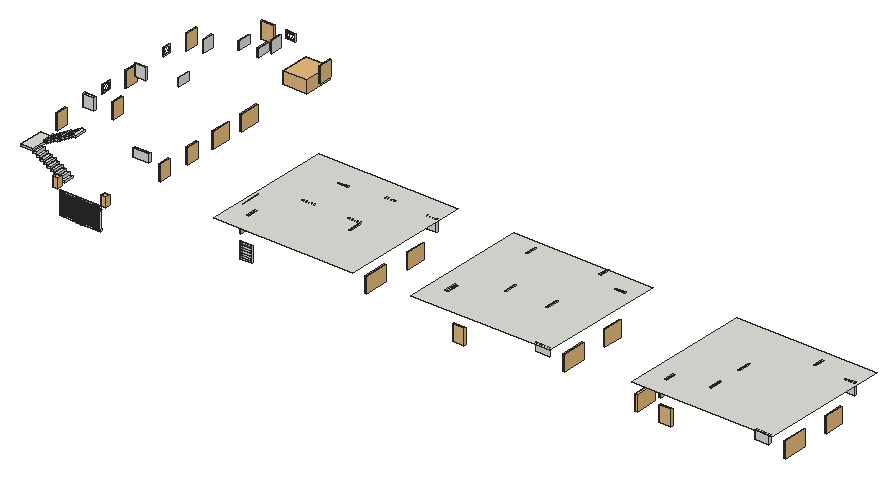
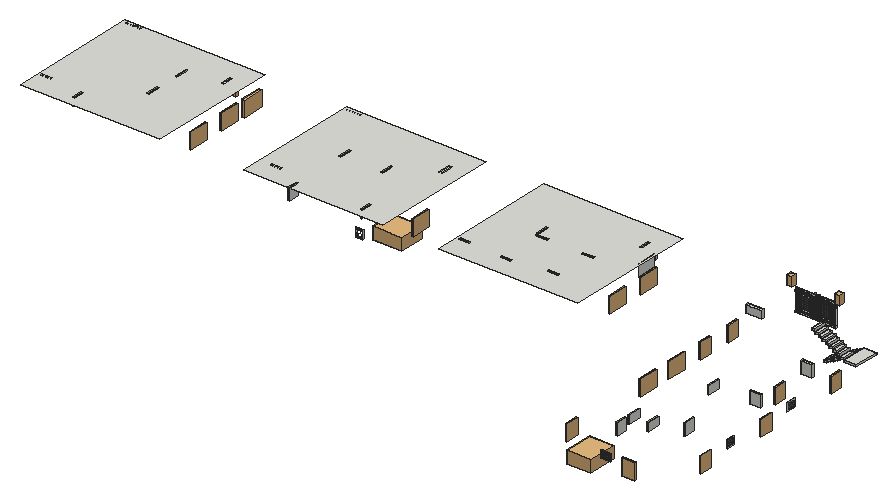
# SketchUp Ruby script. Lengths in inches.
U = 1.inch
M = Sketchup.active_model
def pt(a) = Geom::Point3d.new(a.map { |v| v * U })
def face(e, loops, mat)
  f = e.add_face(loops[0].map { |a| pt(a) })
  loops[1..].each { |l| e.add_face(l.map { |a| pt(a) }).erase! }
  f.material = f.back_material = mat if mat
  f
end
# faces: each face lists its corners as indices into pts; further lists are holes
def faces(e, pts, list, mat = nil) = list.each { |f| face(e, (f[0].is_a?(Array) ? f : [f]).map { |l| l.map { |i| pts[i] } }, mat) }
# xy, xz, yz: faces in a plane at the given z, y or x. An outline is a flat list of corners, or four numbers for a rectangle; further outlines are holes
def ring(l) = l.size == 4 ? [[l[0], l[1]], [l[2], l[1]], [l[2], l[3]], [l[0], l[3]]] : l.each_slice(2).to_a
def flat(e, list, mat, &to3) = list.each { |f| face(e, (f[0].is_a?(Array) ? f : [f]).map { |l| ring(l).map { |u, v| to3.(u, v) } }, mat) }
def xy(e, z, list, mat = nil) = flat(e, list, mat) { |x, y| [x, y, z] }
def xz(e, y, list, mat = nil) = flat(e, list, mat) { |x, z| [x, y, z] }
def yz(e, x, list, mat = nil) = flat(e, list, mat) { |y, z| [x, y, z] }
def lines(e, pts, list) = list.each { |a, b| e.add_line(pt(pts[a]), pt(pts[b])) }
# prism: a flat outline (further loops are holes) pulled along v
def prism(e, loops, v, mat = nil)
  f = face(e, loops, mat); d = Geom::Vector3d.new(v.map { |x| x * U })
  f.pushpull(f.normal.samedirection?(d) ? d.length : -d.length)
end
def box(e, o, s, mat = nil) = prism(e, [[o, [o[0] + s[0], o[1], o[2]], [o[0] + s[0], o[1] + s[1], o[2]], [o[0], o[1] + s[1], o[2]]]], [0, 0, s[2]], mat)
def at(x, y, z, deg = 0) = Geom::Transformation.translation(pt([x, y, z])) * Geom::Transformation.rotation(ORIGIN, Z_AXIS, deg.degrees)
def axes(o, x, y, z) = Geom::Transformation.new([*x, 0, *y, 0, *z, 0, *pt(o).to_a, 1])
def part(name) = M.definitions.add(name)
# library, detail: a bought-in or finely detailed component or shape, given as its bounding box
def library(name, o, s) = part(name).tap { |d| box(d.entities, o, s) }
def detail(e, o, s) = box(e.add_group.entities, o, s)
def put(e, d, t, mat = nil) = e.add_instance(d, t).tap { |i| i.material = mat if mat }
def group(e, t, mat = nil) = e.add_group.tap { |g| g.transformation = t; g.material = mat if mat }.entities
root = M.entities
M.materials.add("[Color_000]").color = [255, 255, 255]
M.materials.add("[Color_C20]").color = [102, 91, 81]
M.materials.add("[Translucent_Glass_Gray]").color = [128, 128, 128]
M.materials["[Translucent_Glass_Gray]"].alpha = 0.5
c1 = library("Untitled+(2)",[-25.65,-58.99,0],[75.48,89.46,37.24])
c2 = library("Gate pull handle",[-0.01,0,0],[1.26,2.875,48])
c3 = part("Gate slat")
xy(c3.entities,0,[[0.39,114.16,6.3,114.17]])
xy(c3.entities,0,[[0.39,0,6.3,114.16]],"[Color_C20]")
xy(c3.entities,0.39,[[0.39,0,0.79,114.17],[0.98,0,2.07,114.17],[2.36,0,3.2,114.17],[3.59,0,4.37,114.17],[4.56,0,5.71,114.17],
  [5.91,0,6.3,114.17]],"[Color_C20]")
xy(c3.entities,0.79,[[0.39,0,0.79,114.17],[0.98,0,2.07,114.17],[2.36,0,3.2,114.17],[3.59,0,4.37,114.17],[4.56,0,5.71,114.17],
  [5.91,0,6.3,114.17]],"[Color_C20]")
xy(c3.entities,0.99,[[1.13,0,1.21,114.16],[1.87,0,1.94,114.16],[2.61,0,2.68,114.16],[3.35,0,3.42,114.16],[4.08,0,4.16,114.16],
  [4.82,0,4.9,114.16],[5.5625,0,5.63,114.16],[6.3,0,6.37,114.16]],"[Color_C20]")
xy(c3.entities,1.18,[[0.39,114.16,3.35,114.17],[3.35,114.16,6.3,114.17]])
xy(c3.entities,1.18,[[0.39,0,1.13,114.16],[1.21,0,1.87,114.16],[1.94,0,2.61,114.16],[2.68,0,3.35,114.16],[3.42,0,4.08,114.16],
  [4.16,0,4.82,114.16],[4.9,0,5.5625,114.16],[5.63,0,6.3,114.16]],"[Color_C20]")
xz(c3.entities,0,[[[0.39,0,6.3,0,6.3,0.39,5.91,0.39,5.91,0.79,6.3,0.79,6.3,1.18,5.63,1.18,5.63,0.99,5.5625,0.99,5.5625,1.18,4.9,1.18,4.9,0.99,4.82,0.99,4.82,1.18,4.16,1.18,4.16,0.99,4.08,0.99,4.08,1.18,3.42,1.18,3.42,0.99,3.35,0.99,3.35,1.18,2.68,1.18,2.68,0.99,2.61,0.99,2.61,1.18,1.94,1.18,1.94,0.99,1.87,0.99,1.87,1.18,1.21,1.18,1.21,0.99,1.13,0.99,1.13,1.18,0.39,1.18,0.39,0.79,0.79,0.79,0.79,0.39,0.39,0.39],[4.56,0.39,5.71,0.79],[0.98,0.39,2.07,0.79],[2.36,0.39,3.2,0.79],[3.59,0.39,4.37,0.79]],[6.3,0.99,6.37,1.18]],"[Color_C20]")
xz(c3.entities,114.16,[[1.13,0.99,1.21,1.18],[1.87,0.99,1.94,1.18],[2.61,0.99,2.68,1.18],[3.35,0.99,3.42,1.18],[4.08,0.99,4.16,1.18],
  [4.82,0.99,4.9,1.18],[5.5625,0.99,5.63,1.18]],"[Color_C20]")
xz(c3.entities,114.17,[[[0.39,0,0.39,0.39,0.79,0.39,0.79,0.79,0.39,0.79,0.39,1.18,6.3,1.18,6.3,0.79,5.91,0.79,5.91,0.39,6.3,0.39,6.3,0],[4.56,0.39,5.71,0.79],[0.98,0.39,2.07,0.79],[2.36,0.39,3.2,0.79],[3.59,0.39,4.37,0.79]]],"[Color_C20]")
yz(c3.entities,0.39,[[114.16,0,114.17,0.39],[114.16,0.79,114.17,1.18]])
yz(c3.entities,0.39,[[0,0,114.16,0.39],[0,0.79,114.16,1.18]],"[Color_C20]")
yz(c3.entities,0.79,[[0,0.39,114.17,0.79]],"[Color_C20]")
yz(c3.entities,0.98,[[0,0.39,114.17,0.79]],"[Color_C20]")
yz(c3.entities,1.13,[[0,0.99,114.16,1.18]],"[Color_C20]")
yz(c3.entities,1.21,[[0,0.99,114.16,1.18]],"[Color_C20]")
yz(c3.entities,1.87,[[0,0.99,114.16,1.18]],"[Color_C20]")
yz(c3.entities,1.94,[[0,0.99,114.16,1.18]],"[Color_C20]")
yz(c3.entities,2.07,[[0,0.39,114.17,0.79]],"[Color_C20]")
yz(c3.entities,2.36,[[0,0.39,114.17,0.79]],"[Color_C20]")
yz(c3.entities,2.61,[[0,0.99,114.16,1.18]],"[Color_C20]")
yz(c3.entities,2.68,[[0,0.99,114.16,1.18]],"[Color_C20]")
yz(c3.entities,3.2,[[0,0.39,114.17,0.79]],"[Color_C20]")
yz(c3.entities,3.35,[[0,0.99,114.16,1.18]],"[Color_C20]")
yz(c3.entities,3.42,[[0,0.99,114.16,1.18]],"[Color_C20]")
yz(c3.entities,3.59,[[0,0.39,114.17,0.79]],"[Color_C20]")
yz(c3.entities,4.08,[[0,0.99,114.16,1.18]],"[Color_C20]")
yz(c3.entities,4.16,[[0,0.99,114.16,1.18]],"[Color_C20]")
yz(c3.entities,4.37,[[0,0.39,114.17,0.79]],"[Color_C20]")
yz(c3.entities,4.56,[[0,0.39,114.17,0.79]],"[Color_C20]")
yz(c3.entities,4.82,[[0,0.99,114.16,1.18]],"[Color_C20]")
yz(c3.entities,4.9,[[0,0.99,114.16,1.18]],"[Color_C20]")
yz(c3.entities,5.5625,[[0,0.99,114.16,1.18]],"[Color_C20]")
yz(c3.entities,5.63,[[0,0.99,114.16,1.18]],"[Color_C20]")
yz(c3.entities,5.71,[[0,0.39,114.17,0.79]],"[Color_C20]")
yz(c3.entities,5.91,[[0,0.39,114.17,0.79]],"[Color_C20]")
yz(c3.entities,6.3,[[114.16,0,114.17,0.39],[114.16,0.79,114.17,1.18]])
yz(c3.entities,6.3,[[0,0,114.16,0.39],[0,0.79,114.16,0.99],[0,0.99,114.16,1.18]],"[Color_C20]")
yz(c3.entities,6.37,[[0,0.99,114.16,1.18]],"[Color_C20]")
p = [[0,0,0],[0.39,0,0]]
lines(c3.entities,p,[[0,1]])
c4 = part("Vertical gate panel")
put(c4.entities,c3,axes([0,1.18,0],[3.67755,0,0],[0,0,2.40086],[0,-1,0]))
put(c4.entities,c3,axes([21.72,1.18,0],[3.67755,0,0],[0,0,2.40086],[0,-1,0]))
c5 = part("Group\#1")
prism(c5.entities,[[[0,0,0],[0,31.5,0],[11,31.5,0],[11,0,0],[2,0,0]]],[0,0,6])
c6 = library("Window with transom",[0,0,0],[5.2,55.12,70.87])
c7 = part("Group\#259")
p = [[0,43.31,5.11],[2.95,43.31,0],[2.95,0,0],[0,0,5.11]]
faces(c7.entities,p,[[0,1,2,3]],"[Translucent_Glass_Gray]")
c8 = part("Vwntilation+window (1)")
put(c8.entities,c7,at(43.48,1.97,32.29))
put(c8.entities,c7,at(43.48,1.97,26.38))
put(c8.entities,c7,at(43.48,1.97,20.48))
put(c8.entities,c7,at(43.48,1.97,14.57))
put(c8.entities,c7,at(43.48,1.97,8.67))
put(c8.entities,c7,at(43.48,1.97,2.76))
g1 = group(c8.entities,at(43.48,0,0))
prism(g1,[[[1.97,47.24,39.37],[1.97,0,39.37],[1.97,0,0],[1.97,47.24,0]],[[1.97,45.28,1.97],[1.97,1.97,1.97],[1.97,1.97,37.4],[1.97,45.28,37.4]]],[-1.97,0,0])
c9 = part("Group\#3")
box(c9.entities,[0,0,0],[11,37.5,6])
c10 = library("Group\#257",[0,0,0],[26.45,25.63,49.07])
xy(root,1.13,[[[260.49,22.66,324.4,26.05],[262.38,24.13,262.49,24.15,262.6,24.19,262.69,24.26,262.76,24.36,262.81,24.46,262.82,24.58,262.81,24.69,262.76,24.8,262.69,24.89,262.6,24.97,262.49,25.01,262.38,25.02,262.26,25.01,262.15,24.97,262.0625,24.89,261.99,24.8,261.95,24.69,261.93,24.58,261.95,24.46,261.99,24.36,262.0625,24.26,262.15,24.19,262.26,24.15]],[[324.65,22.66,387.35,25.83],[386.67,24.04,386.79,24.05,386.9,24.09,386.99,24.16,387.06,24.24,387.1,24.34,387.12,24.45,387.1,24.56,387.06,24.66,386.99,24.75,386.9,24.8125,386.79,24.85,386.67,24.87,386.56,24.85,386.45,24.8125,386.36,24.75,386.29,24.66,386.24,24.56,386.23,24.45,386.24,24.34,386.29,24.24,386.36,24.16,386.45,24.09,386.56,24.05]]],"[Color_000]")
xy(root,4.67,[[276.34,22.66,277.85,23.22],[277.85,22.66,309.42,23.22],[309.42,22.66,310.93,23.22],[338.12,22.66,339.63,23.18],[339.63,22.66,371.2,23.18],
  [371.2,22.66,372.71,23.18]])
xy(root,4.67,[[266.41,22.66,271.38,26.05],[271.38,22.66,276.34,26.05],[310.93,22.66,320.86,23.22],[328.1875,22.66,338.12,23.18],[372.71,22.66,377.67,25.83],
  [377.67,22.66,382.64,25.83],[328.1875,23.18,338.12,25.83],[339.63,23.18,371.2,25.83],[277.85,23.22,309.42,26.05],[310.93,23.22,320.86,26.05]],"[Color_000]")
xy(root,6,[[260.49,22.66,262.88,26.05],[386.17,22.66,387.35,25.83]],"[Color_000]")
xy(root,14.6,[[277.85,22.66,309.42,26.05],[339.63,22.66,371.2,25.83]],"[Color_000]")
xy(root,16.11,[[277.85,22.66,309.42,26.05],[339.63,22.66,371.2,25.83]],"[Color_000]")
xy(root,56.27,[[277.85,22.66,309.42,26.05],[339.63,22.66,371.2,25.83]],"[Color_000]")
xy(root,57.78,[[277.85,22.66,309.42,26.05],[339.63,22.66,371.2,25.83]],"[Color_000]")
xy(root,58.06,[[386.17,23.78,387.29,24.97],[261.76,23.86,262.88,25.14]],"[Color_000]")
xy(root,60.46,[[386.17,23.78,387.29,24.97],[261.76,23.86,262.88,25.14]],"[Color_000]")
xy(root,60.57,[[386.17,23.78,387.29,24.97],[387.29,23.78,389.6,24.97],[259.45,23.86,261.76,25.14],[261.76,23.86,262.88,25.14]],"[Color_000]")
xy(root,61.29,[[386.17,23.78,387.29,24.97],[387.29,23.78,389.6,24.97],[259.45,23.86,261.76,25.14],[261.76,23.86,262.88,25.14]],"[Color_000]")
xy(root,61.41,[[386.17,23.78,387.29,24.97],[261.76,23.86,262.88,25.14]],"[Color_000]")
xy(root,63.71,[[386.17,23.78,387.29,24.97],[261.76,23.86,262.88,25.14]],"[Color_000]")
xy(root,67.71,[[266.41,22.66,271.38,26.05],[271.38,22.66,276.34,26.05],[277.85,22.66,309.42,26.05],[310.93,22.66,320.86,26.05],[328.1875,22.66,338.12,25.83],
  [339.63,22.66,371.2,25.83],[372.71,22.66,377.67,25.83],[377.67,22.66,382.64,25.83]],"[Color_000]")
xy(root,71.24,[[262.88,22.66,324.4,26.05],[324.65,22.66,386.17,25.83]],"[Color_000]")
xy(root,120,[[692.13,78.48,1123.13,483.48],[1300.75,78.48,1731.75,474.48],[1983.63,78.48,2414.63,483.48]])
xz(root,22.66,[[[260.49,1.13,324.4,1.13,324.4,71.24,262.88,71.24,262.88,6,260.49,6],[266.41,4.67,320.86,67.71]],[[324.65,1.13,387.35,1.13,387.35,6,386.17,6,386.17,71.24,324.65,71.24],[328.1875,4.67,382.64,67.71]],[276.34,4.67,277.85,14.6],[309.42,4.67,310.93,14.6],[338.12,4.67,339.63,14.6],
  [371.2,4.67,372.71,14.6],[276.34,14.6,310.93,14.6,310.93,57.78,276.34,57.78,276.34,56.27,309.42,56.27,309.42,16.11,277.85,16.11,277.85,56.27,276.34,56.27],[338.12,14.6,372.71,14.6,372.71,56.27,371.2,56.27,371.2,16.11,339.63,16.11,339.63,56.27,372.71,56.27,372.71,57.78,338.12,57.78],[276.34,57.78,277.85,67.71],[309.42,57.78,310.93,67.71],
  [338.12,57.78,339.63,67.71],[371.2,57.78,372.71,67.71]],"[Color_000]")
xz(root,23.78,[[386.17,58.06,387.29,60.46],[386.17,60.57,389.6,61.29],[386.17,61.41,387.29,63.71]],"[Color_000]")
xz(root,23.86,[[261.76,58.06,262.88,60.46],[259.45,60.57,262.88,61.29],[261.76,61.41,262.88,63.71]],"[Color_000]")
xz(root,24.97,[[386.17,58.06,387.29,60.46],[386.17,60.57,387.29,60.85],[387.29,60.57,387.29,60.85,386.17,60.85,386.17,61.29,389.6,61.29,389.6,60.57],[386.17,61.41,387.29,63.71]],"[Color_000]")
xz(root,25.14,[[261.76,58.06,262.88,60.46],[259.45,60.57,259.45,61.29,262.88,61.29,262.88,60.85,261.76,60.85,261.76,60.57],[261.76,60.57,262.88,60.85],[261.76,61.41,262.88,63.71]],"[Color_000]")
xz(root,25.83,[[[324.65,1.13,324.65,71.24,386.17,71.24,386.17,6,387.35,6,387.35,1.13],[339.63,16.11,371.2,56.27],[372.71,4.67,382.64,67.71],[328.1875,4.67,338.12,67.71],[339.63,57.78,371.2,67.71],[339.63,4.67,371.2,14.6]]],"[Color_000]")
xz(root,26.05,[[[260.49,1.13,260.49,6,262.88,6,262.88,71.24,324.4,71.24,324.4,1.13],[277.85,16.11,309.42,56.27],[266.41,4.67,276.34,67.71],[310.93,4.67,320.86,67.71],[277.85,57.78,309.42,67.71],[277.85,4.67,309.42,14.6]]],"[Color_000]")
xz(root,87.48,[[1679.75,96,1722.75,120]])
yz(root,259.45,[[23.86,60.57,25.14,61.29]],"[Color_000]")
yz(root,260.49,[[22.66,1.13,26.05,6]],"[Color_000]")
yz(root,261.76,[[23.86,58.06,25.14,60.46],[23.86,61.41,25.14,63.71]],"[Color_000]")
yz(root,262.88,[[[22.66,6,26.05,71.24],[23.86,58.06,25.14,60.46],[23.86,61.41,25.14,63.71],[23.86,60.57,25.14,61.29]]],"[Color_000]")
yz(root,266.41,[[22.66,4.67,26.05,67.71]],"[Color_000]")
yz(root,276.34,[[22.66,4.67,26.05,14.6],[22.66,14.6,26.05,56.27],[22.66,56.27,26.05,57.78],[22.66,57.78,26.05,67.71]],"[Color_000]")
yz(root,277.85,[[22.66,4.67,26.05,14.6],[22.66,16.11,26.05,56.27],[22.66,57.78,26.05,67.71]],"[Color_000]")
yz(root,309.42,[[22.66,4.67,26.05,14.6],[22.66,16.11,26.05,56.27],[22.66,57.78,26.05,67.71]],"[Color_000]")
yz(root,310.93,[[22.66,4.67,26.05,14.6],[22.66,14.6,26.05,57.78],[22.66,57.78,26.05,67.71]],"[Color_000]")
yz(root,320.86,[[22.66,4.67,26.05,67.71]],"[Color_000]")
yz(root,324.4,[[22.66,1.13,26.05,71.24]],"[Color_000]")
yz(root,324.65,[[22.66,1.13,25.83,71.24]],"[Color_000]")
yz(root,328.1875,[[22.66,4.67,25.83,67.71]],"[Color_000]")
yz(root,338.12,[[22.66,4.67,25.83,14.6],[22.66,14.6,25.83,57.78],[22.66,57.78,25.83,67.71]],"[Color_000]")
yz(root,339.63,[[22.66,4.67,25.83,14.6],[22.66,16.11,25.83,56.27],[22.66,57.78,25.83,67.71]],"[Color_000]")
yz(root,371.2,[[22.66,4.67,25.83,14.6],[22.66,16.11,25.83,56.27],[22.66,57.78,25.83,67.71]],"[Color_000]")
yz(root,372.71,[[22.66,4.67,25.83,14.6],[22.66,14.6,25.83,56.27],[22.66,56.27,25.83,57.78],[22.66,57.78,25.83,67.71]],"[Color_000]")
yz(root,382.64,[[22.66,4.67,25.83,67.71]],"[Color_000]")
yz(root,386.17,[[[22.66,6,25.83,71.24],[23.78,58.06,23.78,60.46,24.97,60.46,24.97,60.57,23.78,60.57,23.78,61.29,24.97,61.29,24.97,58.06],[23.78,61.41,24.97,63.71]]],"[Color_000]")
yz(root,387.29,[[23.78,58.06,24.97,60.46],[23.78,61.41,24.97,63.71]],"[Color_000]")
yz(root,387.35,[[22.66,1.13,25.83,6]],"[Color_000]")
yz(root,701.13,[[178.48,84,239.48,120]])
p = [[373.33,23.18,4.67],[372.71,23.18,4.67],[375.83,23.18,67.7],[339.63,23.18,67.7],[371.19,23.18,58.15],[371.19,23.18,16.11],
  [273.22,23.22,67.7],[309.42,23.22,67.7],[275.72,23.22,4.67],[276.34,23.22,4.67],[277.86,23.22,58.15],[277.86,23.22,16.11],
  [324.4,22.66,1.13],[324.65,22.66,1.13],[262.88,25.14,60.57],[262.88,25.14,60.46]]
lines(root,p,[[0,1],[2,3],[4,5],[6,7],[8,9],[10,11],[12,13],[14,15]])
put(root,c1,at(303.23,921.85,0.9))
put(root,c2,axes([331.23,19.9,1.41],[-0.989,0,0],[0,0.96118,0],[0,0,1.45482]))
put(root,c2,axes([317.82,19.7,1.41],[0.989,0,0],[0,1.03,0],[0,0,1.45482]))
put(root,c4,axes([339.63,23.18,4.33],[0,0,0.23456],[0,0.21463,0],[0.11517,0,0]))
put(root,c4,axes([309.42,23.22,4.33],[0,0,0.23456],[0,0.23,0],[-0.11517,0,0]))
put(root,c3,axes([333.52,23.4375,4.67],[-0.84584,0,0],[0,0,0.5522],[0,-0.21463,0]))
put(root,c3,axes([383.03,23.4375,4.67],[-0.84584,0,0],[0,0,0.5522],[0,-0.21463,0]))
put(root,c3,axes([378.03,23.4375,4.67],[-0.84584,0,0],[0,0,0.5522],[0,-0.21463,0]))
put(root,c3,axes([338.51,23.4375,4.67],[-0.84584,0,0],[0,0,0.5522],[0,-0.21463,0]))
put(root,c3,axes([266.02,23.49,4.67],[0.84584,0,0],[0,0,0.5522],[0,-0.23,0]))
put(root,c3,axes([271.02,23.49,4.67],[0.84584,0,0],[0,0,0.5522],[0,-0.23,0]))
put(root,c3,axes([310.54,23.49,4.67],[0.84584,0,0],[0,0,0.5522],[0,-0.23,0]))
put(root,c3,axes([315.53,23.49,4.67],[0.84584,0,0],[0,0,0.5522],[0,-0.23,0]))
put(root,c1,at(1342.19,338.62,5.79,90))
put(root,c5,at(166,148.42,6))
put(root,c5,at(155,148.42,12))
put(root,c4,axes([339.625,23.18,15.98],[0,0,0.22998],[0,0.21463,0],[0.11517,0,0]))
put(root,c4,axes([309.43,23.22,15.98],[0,0,0.22998],[0,0.23,0],[-0.11517,0,0]))
put(root,c5,at(144,148.42,18))
put(root,c5,at(133,148.42,24))
put(root,c4,axes([339.625,23.18,25.97],[0,0,0.22998],[0,0.21463,0],[0.11517,0,0]))
put(root,c4,axes([309.43,23.22,25.97],[0,0,0.22998],[0,0.23,0],[-0.11517,0,0]))
put(root,c5,at(122,148.42,30))
put(root,c4,axes([339.63,23.18,35.96],[0,0,0.22998],[0,0.21463,0],[0.11517,0,0]))
put(root,c4,axes([309.42,23.22,35.96],[0,0,0.22998],[0,0.23,0],[-0.11517,0,0]))
put(root,c6,axes([1300.71,298.48,35.96],[1,0,0],[0,1.08857,0],[0,0,0.67733]))
put(root,c6,axes([1114.09,134.48,35.96],[1,0,0],[0,1.33894,0],[0,0,0.67733]))
put(root,c6,axes([1123.13,290.48,35.96],[-0.73939,0,0],[0,1.08857,0],[0,0,0.67733]))
put(root,c6,axes([29.96,564.92,35.96],[1,0,0],[0,0.70757,0],[0,0,0.67733]))
put(root,c6,axes([29.96,797.29,35.96],[1,0,0],[0,0.70757,0],[0,0,0.67733]))
put(root,c6,axes([380.96,874.91,35.96],[1,0,0],[0,0.70757,0],[0,0,0.67733]))
put(root,c6,axes([380.96,569.64,35.96],[1,0,0],[0,1.10381,0],[0,0,0.67733]))
put(root,c6,axes([380.96,459.92,35.96],[1,0,0],[0,1.10381,0],[0,0,0.67733]))
put(root,c6,axes([380.96,361.31,35.96],[1,0,0],[0,0.66512,0],[0,0,0.67733]))
put(root,c6,axes([380.96,255.61,35.96],[1,0,0],[0,0.66512,0],[0,0,0.67733]))
put(root,c6,axes([692.15,178.46,35.96],[1,0,0],[0,1.10671,0],[0,0,0.67733]))
put(root,c6,axes([692.15,298.48,35.96],[1,0,0],[0,1.10671,0],[0,0,0.67733]))
put(root,c6,axes([1987.4375,178.48,36],[1,0,0],[0,1.10671,0],[0,0,0.67733]))
put(root,c6,axes([1987.4375,298.48,36],[1,0,0],[0,1.08857,0],[0,0,0.67733]))
put(root,c6,axes([1983.63,88.48,36],[1.73182,0,0],[0,1.23371,0],[0,0,0.67733]))
put(root,c8,axes([773.13,142.97,36],[0,-1.3889,0],[0.762,0,0],[0,0,1.2192]))
put(root,c6,axes([30,296.72,36],[1,0,0],[0,0.65314,0],[0,0,0.67733]))
put(root,c6,axes([174,957.23,36],[0,1,0],[-0.70757,0,0],[0,0,0.67733]))
put(root,c6,axes([100.5,423.92,36],[1.23,0,0],[0,0.64389,0],[0,0,0.67733]))
put(root,c6,axes([1726.56,134.48,36],[1,0,0],[0,1.34257,0],[0,0,0.67733]))
put(root,c6,axes([1726.56,290.48,36],[1,0,0],[0,1.08857,0],[0,0,0.67733]))
put(root,c6,axes([2409.18,290.7,36],[1.05,0,0],[0,1.08458,0],[0,0,0.67733]))
put(root,c6,axes([2409.18,134.48,36],[1.05,0,0],[0,1.34257,0],[0,0,0.67733]))
put(root,c6,axes([1461.75,83.28,36],[0,1,0],[-0.65552,0,0],[0,0,0.67733]))
put(root,c6,axes([2100.63,83.28,36],[0,1,0],[-0.65552,0,0],[0,0,0.67733]))
put(root,c5,at(111,148.42,36))
put(root,c5,at(100,148.42,42))
put(root,c4,axes([339.63,23.18,45.95],[0,0,0.22998],[0,0.21463,0],[0.11517,0,0]))
put(root,c4,axes([309.42,23.22,45.95],[0,0,0.22998],[0,0.23,0],[-0.11517,0,0]))
put(root,c5,at(89,148.42,48))
put(root,c5,at(78,148.42,54))
put(root,c4,axes([339.63,23.18,57.18],[0,0,0.23456],[0,0.21463,0],[0.11517,0,0]))
put(root,c4,axes([309.42,23.22,57.18],[0,0,0.23456],[0,0.23,0],[-0.11517,0,0]))
put(root,c8,axes([94.49,732.63,60],[-1.3889,0,0],[0,-0.508,0],[0,0,0.6096]))
put(root,c8,axes([94.49,501.82,60],[-1.3889,0,0],[0,-0.635,0],[0,0,0.6096]))
g2 = group(root,at(39,148.42,60))
box(g2,[0,0,0],[39,78,6])
put(root,c8,axes([1359.6,538.97,60],[0,-1.3889,0],[0.51054,0,0],[0,0,0.6096]))
put(root,c8,axes([238.5,934.1,62.25],[0,0.61,0],[-0.635,0,0],[0,0,0.55235]))
put(root,c9,at(78,188.92,66))
put(root,c9,at(89,188.92,72))
put(root,c10,axes([241.95,20.69,74.85],[0.58,0,0],[0,0.58,0],[0,0,0.58]))
put(root,c10,axes([390.15,20.69,74.85],[0.58,0,0],[0,0.58,0],[0,0,0.58]))
put(root,c9,at(100,188.92,78))
g3 = group(root,at(121.5,749.42,0))
box(g3,[0,0,84],[4.5,33,36])
put(root,c9,at(111,188.92,84))
g4 = group(root,at(63,359.92,0))
box(g4,[0,0,84],[33,9,36])
g5 = group(root,at(67.5,555.92,0))
box(g5,[0,0,84],[33,4.5,36])
g6 = group(root,at(250.5,849.92,0))
box(g6,[0,0,84],[4.5,33,36])
g7 = group(root,at(1348.75,151.48,0))
box(g7,[0,0,84],[9,36,36])
g8 = group(root,at(744.13,141.48,0))
box(g8,[0,0,84],[5,31,36])
g9 = group(root,at(1084.13,410.48,0))
box(g9,[0,0,84],[30,5,36])
g10 = group(root,at(951.13,416.48,0))
box(g10,[0,0,84],[30,5,36])
g11 = group(root,at(803.13,281.48,0))
box(g11,[0,0,84],[36,5,36])
g12 = group(root,at(2035.63,141.48,0))
box(g12,[0,0,84],[5,31,36])
g13 = group(root,at(2375.63,410.48,0))
box(g13,[0,0,84],[30,5,36])
g14 = group(root,at(1589.75,444.48,0))
box(g14,[0,0,84],[5,30,36])
g15 = group(root,at(818.13,400.48,0))
box(g15,[0,0,84.07],[31,5,35.93])
put(root,c9,at(122,188.92,90))
g16 = group(root,at(192,564.92,0))
box(g16,[0,0,96],[4.5,39,24])
g17 = group(root,at(192,797.42,0))
box(g17,[0,0,96],[4.5,39,24])
g18 = group(root,at(250.5,797.42,0))
box(g18,[0,0,96],[4.5,39,24])
g19 = group(root,at(2362.63,78.48,0))
box(g19,[0,0,96],[43,9,24])
put(root,c9,at(133,188.92,96))
g20 = group(root,at(324,226.42,0))
box(g20,[0,0,96],[48,9,24])
g21 = group(root,at(1589.75,239.48,0))
box(g21,[0,0,96],[5,39,24])
g22 = group(root,at(1461.75,239.48,0))
box(g22,[0,0,96],[5,36,24])
g23 = group(root,at(1385.75,416.98,0))
box(g23,[0,0,96],[5,33,24])
g24 = group(root,at(1666.75,410.48,0))
box(g24,[0,0,96],[30,5,24])
g25 = group(root,at(945.13,281.48,0))
box(g25,[0,0,96],[36,5,24])
g26 = group(root,at(981.13,239.48,0))
box(g26,[0,0,96],[5,36,24])
g27 = group(root,at(2144.63,176.48,0))
box(g27,[0,0,96],[5,39,24])
g28 = group(root,at(2144.63,286.48,0))
box(g28,[0,0,96],[5,39,24])
g29 = group(root,at(2272.63,421.48,0))
box(g29,[0,0,96],[5,30,24])
put(root,c9,at(144,188.92,102))
put(root,c9,at(155,188.92,108))
put(root,c9,at(166,188.92,114))
